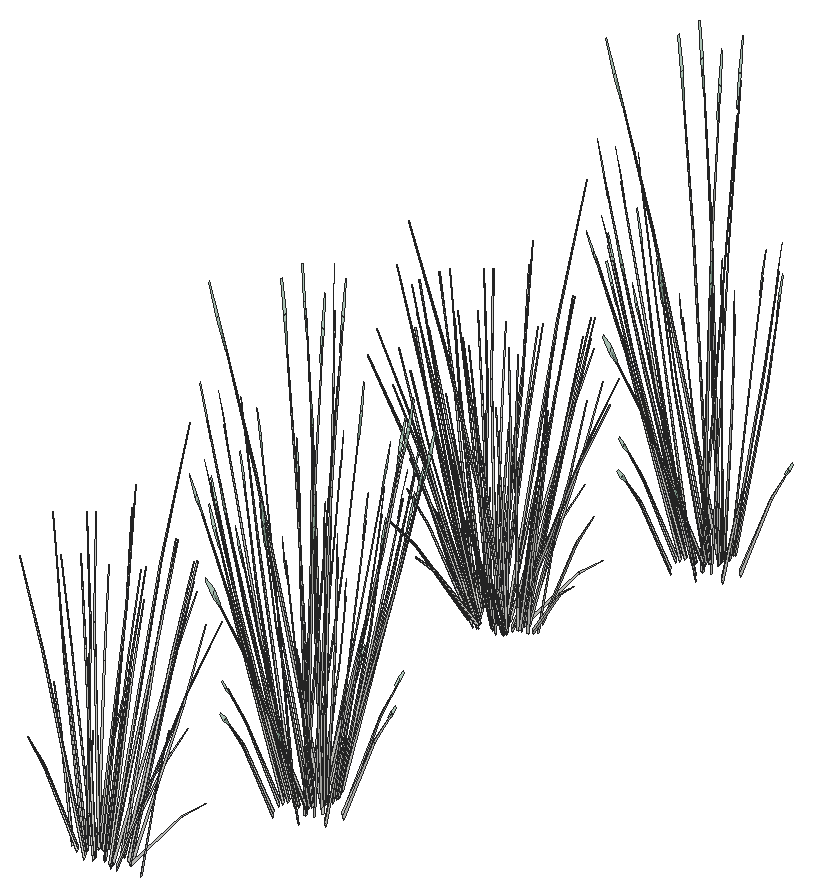
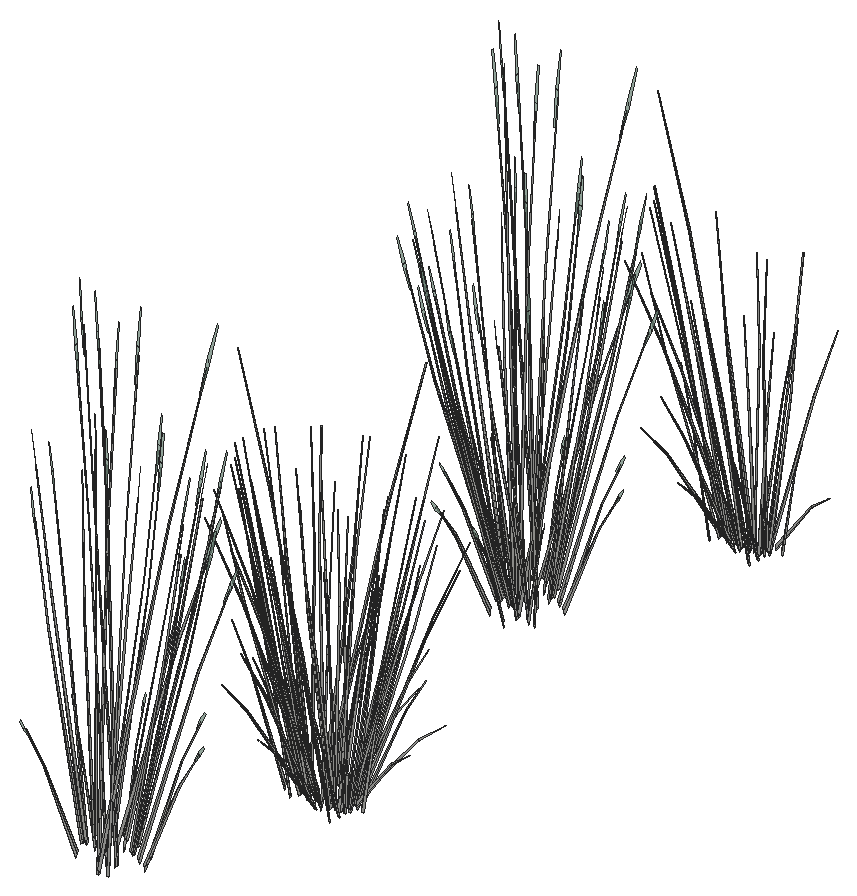
# SketchUp Ruby script. Lengths in inches.
U = 1.inch
M = Sketchup.active_model
def pt(a) = Geom::Point3d.new(a.map { |v| v * U })
def face(e, loops, mat)
  f = e.add_face(loops[0].map { |a| pt(a) })
  loops[1..].each { |l| e.add_face(l.map { |a| pt(a) }).erase! }
  f.material = f.back_material = mat if mat
  f
end
# faces: each face lists its corners as indices into pts; further lists are holes
def faces(e, pts, list, mat = nil) = list.each { |f| face(e, (f[0].is_a?(Array) ? f : [f]).map { |l| l.map { |i| pts[i] } }, mat) }
# xy, xz, yz: faces in a plane at the given z, y or x. An outline is a flat list of corners, or four numbers for a rectangle; further outlines are holes
def ring(l) = l.size == 4 ? [[l[0], l[1]], [l[2], l[1]], [l[2], l[3]], [l[0], l[3]]] : l.each_slice(2).to_a
def flat(e, list, mat, &to3) = list.each { |f| face(e, (f[0].is_a?(Array) ? f : [f]).map { |l| ring(l).map { |u, v| to3.(u, v) } }, mat) }
def xy(e, z, list, mat = nil) = flat(e, list, mat) { |x, y| [x, y, z] }
def xz(e, y, list, mat = nil) = flat(e, list, mat) { |x, z| [x, y, z] }
def yz(e, x, list, mat = nil) = flat(e, list, mat) { |y, z| [x, y, z] }
def lines(e, pts, list) = list.each { |a, b| e.add_line(pt(pts[a]), pt(pts[b])) }
# prism: a flat outline (further loops are holes) pulled along v
def prism(e, loops, v, mat = nil)
  f = face(e, loops, mat); d = Geom::Vector3d.new(v.map { |x| x * U })
  f.pushpull(f.normal.samedirection?(d) ? d.length : -d.length)
end
def box(e, o, s, mat = nil) = prism(e, [[o, [o[0] + s[0], o[1], o[2]], [o[0] + s[0], o[1] + s[1], o[2]], [o[0], o[1] + s[1], o[2]]]], [0, 0, s[2]], mat)
def at(x, y, z, deg = 0) = Geom::Transformation.translation(pt([x, y, z])) * Geom::Transformation.rotation(ORIGIN, Z_AXIS, deg.degrees)
def axes(o, x, y, z) = Geom::Transformation.new([*x, 0, *y, 0, *z, 0, *pt(o).to_a, 1])
def part(name) = M.definitions.add(name)
# library, detail: a bought-in or finely detailed component or shape, given as its bounding box
def library(name, o, s) = part(name).tap { |d| box(d.entities, o, s) }
def detail(e, o, s) = box(e.add_group.entities, o, s)
def put(e, d, t, mat = nil) = e.add_instance(d, t).tap { |i| i.material = mat if mat }
def group(e, t, mat = nil) = e.add_group.tap { |g| g.transformation = t; g.material = mat if mat }.entities
root = M.entities
M.materials.add("LightPink_Translucent").color = [175, 214, 192]
M.materials["LightPink_Translucent"].alpha = 0.75
c1 = part("blade")
p = [[2.15,0.21,22],[0,0.17,0],[0.09,0.45,0],[2.18,0.31,22],[2.29,0.31,22],[0.38,0.45,0],
  [2.48,0.24,33],[2.49,0.24,33],[2.48,0.22,33]]
faces(c1.entities,p,[[0,1,2,3],[4,5,2,3],[6,3,4,7],[8,0,3,6]])
c2 = part("blade with seeds\#1")
put(c2.entities,c1,at(0,0,0))
c3 = part("seeds")
p = [[0.3,-0.1,1.38],[-0.01,-0.03,1.59],[-0.01,-0.03,0.03],[0.14,-0.07,-0.07],[0.29,-0.03,3],[0.15,0.01,3.11]]
faces(c3.entities,p,[[0,1,2,3],[1,0,4,5]],"LightPink_Translucent")
c4 = part("blade with seeds")
put(c4.entities,c1,at(0,0,0))
put(c4.entities,c3,axes([2.4,0.25,30.99],[1.5799,-0.05474,1.17369],[-0.12525,1.92788,0.29478],[-0.07173,-0.02425,1.56792]))
put(root,c2,axes([483.4375,257.72,140.59],[-0.08118,0.04947,1.43516],[0.00691,0.36146,-0.22697],[-0.18608,0.04701,0.1151]))
put(root,c2,axes([488.9,258.875,139.94],[-0.09515,-0.32031,-0.02864],[0.44972,-0.07364,-0.12987],[0.09391,0.02031,0.42837]))
put(root,c2,axes([487.73,258.87,140.85],[0.02662,-0.38751,-0.09976],[0.50399,0.01059,-0.55369],[0.19411,0.02692,0.84132]))
put(root,c2,axes([488.17,258.63,140.59],[0.10664,-0.00644,1.43516],[0.29251,-0.29603,-0.22697],[0.18969,0.03908,0.1151]))
put(root,c2,axes([483.9,258.35,140.6],[-0.12329,-0.35069,0.39379],[0.48364,-0.06086,0.3247],[-0.14254,0.08248,0.81485]))
put(root,c2,axes([483.96,257.86,139.9],[0.17249,-0.0806,1.40588],[0.14522,0.37244,0.11368],[-0.2708,0.08417,0.601]))
put(root,c2,axes([482.53,258.09,140.58],[0.06344,0.01022,1.45516],[0.19627,0.33667,-0.1375],[-0.12987,0.08837,0.25751]))
put(root,c2,axes([483.85,258.41,140.43],[-0.43273,0.05446,-0.29052],[-0.11427,-0.31131,0.37506],[-0.12401,0.08362,0.71765]))
put(root,c2,axes([488.05,258.84,140.43],[0.28286,0.23857,-0.29052],[-0.32298,0.22584,0.37506],[0.1641,0.03436,0.71765]))
put(root,c2,axes([487.94,258.84,140.6],[-0.36656,0.25108,0.39379],[-0.31614,-0.26664,0.3247],[0.17198,0.04631,0.81485]))
put(root,c2,axes([487.07,257.36,140.39],[-0.42958,-0.19798,1.1344],[0.45359,-0.30825,0.48946],[0.1386,0.18577,1.09651]))
put(root,c2,axes([487.04,258.23,139.9],[-0.18466,-0.06565,1.40588],[0.38215,-0.27542,0.11368],[0.23818,0.12424,0.601]))
put(root,c2,axes([483.98,258.2,140.85],[0.45986,0.21011,-0.09976],[-0.26493,0.30427,-0.55369],[-0.12992,0.10577,0.84132]))
put(root,c2,axes([484.6,258.11,139.9],[0.12417,-0.11708,1.40588],[0.31352,0.31602,0.11368],[-0.21504,0.14392,0.601]))
put(root,c2,axes([486.74,259.29,140.85],[0.29624,-0.32616,-0.09976],[0.42901,0.1879,-0.55369],[0.14913,0.09215,0.84132]))
put(root,c2,axes([486.35,259.56,140.58],[0.00147,-0.04613,1.45516],[0.42603,-0.20353,-0.1375],[0.14798,0.07265,0.25751]))
put(root,c2,axes([484.61,259.06,140.6],[-0.354,-0.25999,0.39379],[0.37594,-0.22422,0.3247],[-0.0653,0.12198,0.81485]))
put(root,c2,axes([486.94,259.34,140.6],[-0.49445,0.08745,0.39379],[-0.08581,-0.34303,0.3247],[0.11629,0.1011,0.81485]))
put(root,c2,axes([484.5,258.39,139.9],[0.09256,-0.13097,1.40588],[0.38832,0.27104,0.11368],[-0.17518,0.16893,0.601]))
put(root,c2,axes([484.61,259.13,140.43],[-0.33637,0.20062,-0.29052],[-0.31842,-0.22908,0.37506],[-0.04845,0.11639,0.71765]))
put(root,c2,axes([485.59,259.44,140.6],[-0.36632,0.1295,0.05275],[-0.1793,-0.23615,0.41527],[0.03538,0.1041,0.63322]))
put(root,c2,axes([483.45,259.07,140.59],[-0.01236,0.0754,1.43516],[0.35069,0.26232,-0.22697],[-0.09181,0.12405,0.1151]))
put(root,c2,axes([484.57,258.9,141.15],[0.54637,0.01888,-0.11073],[-0.01493,0.35746,-0.6146],[-0.03795,0.13767,0.93387]))
put(root,c2,axes([485.58,259.3,140.85],[0.48648,-0.17741,-0.09976],[0.23906,0.31487,-0.55369],[0.06419,0.13269,0.84132]))
put(root,c2,axes([484.94,259.04,140.82],[0.35588,0.25603,-0.4653],[-0.37594,0.22422,-0.36041],[-0.05415,0.13008,0.89031]))
put(root,c2,axes([486.28,258.61,139.9],[-0.11364,-0.12234,1.40588],[0.52511,-0.103,0.11368],[0.11868,0.19206,0.601]))
put(root,c2,axes([485.78,259.49,140.43],[-0.14987,0.29303,-0.29052],[-0.43725,-0.08547,0.37506],[0.04009,0.11798,0.71765]))
put(root,c2,axes([485.35,258.67,139.9],[-0.01217,-0.14625,1.40588],[0.52737,0.09702,0.11368],[-0.03262,0.20842,0.601]))
put(root,c2,axes([483.41,259.85,140.58],[0.0564,-0.02301,1.45516],[0.46615,0.15302,-0.1375],[-0.01095,0.12741,0.25751]))
put(root,c2,axes([485.47,260.01,140.59],[0.06302,0.06136,1.43516],[0.50855,0.02411,-0.22697],[0.05114,0.13532,0.1151]))
put(root,c2,axes([484.65,259.42,139.48],[0.01092,-0.19671,1.26617],[0.49126,0.1039,0.17497],[-0.04257,0.20964,0.59789]))
put(root,c4,axes([493.37,274.375,140.21],[0.06442,0.13585,1.61128],[-0.4498,0.04685,0.1261],[-0.05969,-0.29426,0.57588]))
put(root,c4,axes([494.09,273.93,141.7],[0.01072,-0.47777,-0.64651],[0.45152,0.03209,0.07802],[0.04765,-0.2024,0.91455]))
put(root,c4,axes([493.3125,273.17,141.29],[0.12423,-0.3972,-0.32227],[0.36244,0.11585,0.41605],[-0.03323,-0.15992,0.79608]))
put(root,c4,axes([493.125,273.4375,141.43],[-0.40508,-0.12948,-0.465],[0.13885,-0.44393,-0.36018],[-0.03714,-0.17873,0.88973]))
put(root,c4,axes([494,273.78,141.43],[-0.29499,-0.34704,-0.465],[0.31162,-0.30393,-0.36018],[0.04488,-0.17633,0.88973]))
put(root,c4,axes([491.39,272.5625,139.6875],[0.20183,0.19918,1.04523],[-0.31952,0.0786,0.76796],[-0.05721,-0.14394,0.23022]))
put(root,c4,axes([494.28,273.65,141.29],[0.27882,-0.27194,-0.32227],[0.26394,0.31051,0.41605],[0.04016,-0.15777,0.79608]))
put(root,c4,axes([492.27,273.3125,141.29],[-0.06364,-0.41603,-0.32227],[0.36383,-0.10985,0.41605],[-0.09772,-0.11922,0.79608]))
put(root,c4,axes([493.61,272.99,139.6875],[0.03187,0.30513,1.04523],[-0.28077,-0.19355,0.76796],[0.04212,-0.15079,0.23022]))
put(root,c4,axes([492.22,273.65,141.43],[-0.40663,0.12278,-0.465],[-0.07113,-0.46497,-0.36018],[-0.10922,-0.13325,0.88973]))
put(root,c4,axes([494.625,274.76,141.7],[0.21525,-0.40754,-0.64651],[0.37719,0.28963,0.07802],[0.12852,-0.14765,0.91455]))
put(root,c4,axes([494.61,274.57,141.43],[-0.10586,-0.47162,-0.465],[0.4009,-0.0825,-0.36018],[0.11489,-0.12667,0.88973]))
put(root,c4,axes([494.91,274.625,141.29],[0.3587,-0.07382,-0.32227],[0.09472,0.42197,0.41605],[0.10279,-0.11334,0.79608]))
put(root,c4,axes([491.42,274.04,141.29],[-0.23447,-0.32338,-0.32227],[0.26773,-0.30612,0.41605],[-0.13603,-0.04658,0.79608]))
put(root,c4,axes([492.19,275.74,140.2],[-0.17958,0.41302,1.37647],[-0.38687,-0.40462,0.54432],[0.22929,-0.18124,1.15394]))
put(root,c4,axes([495.45,274.16,139.6875],[-0.155,0.24931,1.04523],[-0.09317,-0.36309,0.76796],[0.11912,-0.07769,0.23022]))
put(root,c4,axes([491.67,274.26,142.03],[-0.41193,-0.01244,-0.71763],[0.02767,-0.52368,0.0866],[-0.17451,-0.05527,1.01516]))
put(root,c4,axes([490.51,274.25,139.6875],[0.2648,-0.01237,1.04523],[-0.18886,0.30908,0.76796],[-0.12621,-0.06079,0.23022]))
put(root,c4,axes([491.09,274.08,140.23],[0.22989,0.0105,1.40454],[-0.12143,0.4723,0.19409],[-0.24501,-0.04092,0.66323]))
put(root,c4,axes([491.54,274.37,141.72],[-0.29922,0.34214,-0.51615],[-0.26205,-0.36143,-0.3998],[-0.15203,-0.05206,0.9876]))
put(root,c4,axes([493.05,276.38,139.76],[0.4193,-0.01306,1.28558],[-0.10869,0.59089,0.54432],[-0.22943,-0.13975,1.21348]))
put(root,c4,axes([494.8,275.62,141.43],[0.11164,-0.46982,-0.465],[0.38276,0.16104,-0.36018],[0.1541,-0.04308,0.88973]))
put(root,c4,axes([492.79,275.03,139.64],[-0.40128,-0.23189,0.40713],[0.19312,-0.48183,-0.19594],[0.0925,0,1.30716]))
put(root,c4,axes([494.73,275.79,141.7],[0.3621,-0.22811,-0.64651],[0.2018,0.46957,0.07802],[0.17496,-0.05334,0.91455]))
put(root,c4,axes([492.61,276.15,139.64],[0.02749,0.519,0.40713],[-0.45634,0.04694,-0.19594],[-0.04625,-0.09291,1.30716]))
put(root,c4,axes([495.04,275.84,141.29],[0.34247,0.14409,-0.32227],[-0.09989,0.42037,0.41605],[0.13788,-0.03855,0.79608]))
put(root,c4,axes([491.01,275.17,141.29],[-0.34247,-0.14409,-0.32227],[0.09989,-0.42037,0.41605],[-0.13788,0.03855,0.79608]))
put(root,c4,axes([493.35,275.15,139.64],[-0.02749,-0.519,0.40713],[0.45634,-0.04694,-0.19594],[0.04625,0.09291,1.30716]))
put(root,c4,axes([491.32,275.21,141.7],[-0.3621,0.22811,-0.64651],[-0.2018,-0.46957,0.07802],[-0.17496,0.05334,0.91455]))
put(root,c4,axes([495.76,275.91,139.6875],[-0.25968,0.06131,1.04523],[0.14383,-0.34012,0.76796],[0.13297,0.0366,0.23022]))
put(root,c4,axes([493.17,276.27,139.64],[0.40128,0.23189,0.40713],[-0.19312,0.48183,-0.19594],[-0.0925,0,1.30716]))
put(root,c4,axes([491.25,275.38,141.43],[-0.11164,0.46982,-0.465],[-0.38276,-0.16104,-0.36018],[-0.1541,0.04308,0.88973]))
put(root,c4,axes([493.54,275.77,139.64],[0.37379,-0.28711,0.40713],[0.26322,0.43489,-0.19594],[-0.04625,0.09291,1.30716]))
put(root,c4,axes([494.51,276.64,141.43],[0.29922,-0.34214,-0.465],[0.26205,0.36143,-0.36018],[0.15203,0.05206,0.88973]))
put(root,c4,axes([494.375,276.74,141.7],[0.41193,0.01244,-0.64651],[-0.02767,0.52368,0.07802],[0.17451,0.05527,0.91455]))
put(root,c4,axes([494.62,276.96,141.29],[0.23447,0.32338,-0.32227],[-0.26773,0.30612,0.41605],[0.13603,0.04658,0.79608]))
put(root,c4,axes([491.61,277.04,139.6875],[0.12805,-0.2691,1.04523],[0.13011,0.34747,0.76796],[-0.11021,0.09372,0.23022]))
put(root,c4,axes([491.02,277.08,139.6],[0.01397,-0.30649,0.95605],[0.29664,0.2024,0.52785],[-0.10539,0.12108,0.74993]))
put(root,c4,axes([491.43,276.43,141.43],[0.10586,0.47162,-0.465],[-0.4009,0.0825,-0.36018],[-0.11489,0.12667,0.88973]))
put(root,c4,axes([493.82,277.35,141.43],[0.40663,-0.12278,-0.465],[0.07113,0.46497,-0.36018],[0.10922,0.13325,0.88973]))
put(root,c4,axes([491.72,278.16,140.75],[0.37435,-0.09148,-0.03177],[0.08606,0.43236,-0.14407],[-0.02373,0.09029,0.47519]))
put(root,c4,axes([494.63,277.92,139.6875],[-0.2267,-0.15919,1.04523],[0.30457,-0.13683,0.76796],[0.07632,0.13148,0.23022]))
put(root,c4,axes([493.78,277.69,141.29],[0.06364,0.41603,-0.32227],[-0.36383,0.10985,0.41605],[0.09772,0.11922,0.79608]))
put(root,c4,axes([493.66,277.36,141.7],[0.35138,0.24965,-0.64651],[-0.24972,0.43748,0.07802],[0.12731,0.14906,0.91455]))
put(root,c4,axes([491.77,277.36,141.29],[-0.27882,0.27194,-0.32227],[-0.26394,-0.31051,0.41605],[-0.04016,0.15777,0.79608]))
put(root,c4,axes([492.92,277.5625,141.43],[0.40508,0.12948,-0.465],[-0.13885,0.44393,-0.36018],[0.03714,0.17873,0.88973]))
put(root,c4,axes([492.66,278.68,139.6875],[-0.07352,-0.2953,1.04523],[0.30384,0.139,0.76796],[-0.02079,0.15666,0.23022]))
put(root,c4,axes([492.73,277.84,141.29],[-0.12423,0.3972,-0.32227],[-0.36244,-0.11585,0.41605],[0.03323,0.15992,0.79608]))
put(root,c4,axes([491.95,277.07,141.7],[-0.01072,0.47777,-0.64651],[-0.45152,-0.03209,0.07802],[-0.04765,0.2024,0.91455]))
put(root,c4,axes([492.77,277.48,141.7],[0.19668,0.41997,-0.64651],[-0.40486,0.23405,0.07802],[0.04599,0.20292,0.91455]))
put(root,c2,axes([485.03,306.2,139.9],[0.11364,0.12234,1.40588],[-0.52511,0.103,0.11368],[-0.11868,-0.19206,0.601]))
put(root,c2,axes([485.9,305.39,140.59],[-0.07604,-0.05342,1.43516],[-0.50744,0.03387,-0.22697],[-0.08099,-0.12778,0.1151]))
put(root,c2,axes([488.07,305.77,140.58],[-0.05049,0.0291,1.45516],[-0.49465,-0.09819,-0.1375],[-0.01791,-0.12701,0.25751]))
put(root,c2,axes([488.18,306.05,140.59],[-0.0048,-0.07584,1.43516],[-0.40531,-0.21918,-0.22697],[0.06266,-0.13286,0.1151]))
put(root,c2,axes([486.8,306.42,139.9],[-0.09256,0.13097,1.40588],[-0.38832,-0.27104,0.11368],[0.17518,-0.16893,0.601]))
put(root,c2,axes([486.47,306.03,140.43],[0.14987,-0.29303,-0.29052],[0.43725,0.08547,0.37506],[-0.04009,-0.11798,0.71765]))
put(root,c2,axes([485.375,305.22,140.58],[-0.00927,0.04567,1.45516],[-0.45742,0.16576,-0.1375],[-0.1346,-0.08473,0.25751]))
put(root,c2,axes([486.67,306.22,140.85],[-0.48648,0.17741,-0.09976],[-0.23906,-0.31487,-0.55369],[-0.06419,-0.13269,0.84132]))
put(root,c2,axes([486.53,306.1,140.6],[0.48986,0.09962,0.39379],[-0.16751,0.3275,0.3247],[-0.02944,-0.12879,0.81485]))
put(root,c2,axes([487.68,306.61,140.85],[-0.54637,-0.01888,-0.09976],[0.01493,-0.35746,-0.55369],[0.03795,-0.13767,0.84132]))
put(root,c2,axes([485.21,306.14,140.43],[-0.07678,-0.30692,-0.29052],[0.43892,-0.08104,0.37506],[-0.11789,-0.08795,0.71765]))
put(root,c2,axes([487.64,306.38,140.43],[0.33637,-0.20062,-0.29052],[0.31842,0.22908,0.37506],[0.04845,-0.11639,0.71765]))
put(root,c2,axes([484.27,306.58,139.9],[0.18466,0.06565,1.40588],[-0.38215,0.27542,0.11368],[-0.23818,-0.12424,0.601]))
put(root,c2,axes([485.5,306.08,141.17],[-0.33178,0.3653,-0.11173],[-0.48049,-0.21045,-0.62013],[-0.16702,-0.10321,0.94228]))
put(root,c2,axes([487.64,306.46,140.6],[0.354,0.25999,0.39379],[-0.37594,0.22422,0.3247],[0.0653,-0.12198,0.81485]))
put(root,c2,axes([484.23,305.98,140.59],[-0.10696,-0.00269,1.43516],[-0.34054,0.26896,-0.22697],[-0.1817,-0.05496,0.1151]))
put(root,c2,axes([488.27,307.32,140.85],[-0.45986,-0.21011,-0.09976],[0.26493,-0.30427,-0.55369],[0.12992,-0.10577,0.84132]))
put(root,c2,axes([489.41,307.23,140.58],[-0.06493,-0.00289,1.45516],[-0.26964,-0.31009,-0.1375],[0.10828,-0.10196,0.25751]))
put(root,c2,axes([486.375,308.47,139.45],[0.4296,0.15365,1.24087],[-0.42086,0.33102,0.4907],[-0.18851,-0.19619,1.04025]))
put(root,c2,axes([484.2,306.68,140.43],[-0.28286,-0.23857,-0.29052],[0.32298,-0.22584,0.37506],[-0.1641,-0.03436,0.71765]))
put(root,c2,axes([488.4,307.11,140.43],[0.43273,-0.05446,-0.29052],[0.11427,0.31131,0.37506],[0.12401,-0.08362,0.71765]))
put(root,c2,axes([488.35,307.17,140.6],[0.12329,0.35069,0.39379],[-0.48364,0.06086,0.3247],[0.14254,-0.08248,0.81485]))
put(root,c2,axes([489.65,307.6,140.59],[0.06898,-0.05804,1.43516],[-0.0883,-0.35603,-0.22697],[0.17309,-0.0675,0.1151]))
put(root,c2,axes([483.82,306.21,140.58],[0.03685,0.03803,1.45516],[-0.17767,0.34183,-0.1375],[-0.17994,0.00247,0.25751]))
put(root,c2,axes([484.52,306.65,140.85],[-0.02662,0.38751,-0.09976],[-0.50399,-0.01059,-0.55369],[-0.19411,-0.02692,0.84132]))
put(root,c2,axes([488.29,308.14,140.85],[-0.25013,-0.34504,-0.09976],[0.44394,-0.16956,-0.55369],[0.18708,-0.04552,0.84132]))
put(root,c2,axes([483.88,307.18,139.9],[0.2062,-0.00863,1.40588],[-0.13679,0.37404,0.11368],[-0.29386,-0.02314,0.601]))
put(root,c2,axes([483.79,307.47,140.6],[0.14045,-0.34743,0.39379],[0.46175,0.1188,0.3247],[-0.18159,0.02088,0.81485]))
put(root,c2,axes([483.7,307.51,140.43],[-0.41315,-0.1063,-0.29052],[0.1205,-0.31012,0.37506],[-0.16634,0.02844,0.71765]))
put(root,c2,axes([488.55,308,140.43],[0.41315,0.1063,-0.29052],[-0.1205,0.31012,0.37506],[0.16634,-0.02844,0.71765]))
put(root,c2,axes([487.43,307.62,139.9],[-0.2062,0.00863,1.40588],[0.13679,-0.37404,0.11368],[0.29386,0.02314,0.601]))
put(root,c2,axes([488.46,308.04,140.6],[-0.14045,0.34743,0.39379],[-0.46175,-0.1188,0.3247],[0.18159,-0.02088,0.81485]))
put(root,c2,axes([483.96,307.37,140.85],[0.25013,0.34504,-0.09976],[-0.44394,0.16956,-0.55369],[-0.18708,0.04552,0.84132]))
put(root,c2,axes([489.29,309.16,140.58],[-0.04495,-0.03336,1.45516],[0.09833,-0.35758,-0.1375],[0.17707,-0.02285,0.25751]))
put(root,c2,axes([483.4375,307.71,140.59],[-0.08118,0.04947,1.43516],[0.00691,0.36146,-0.22697],[-0.18608,0.04701,0.1151]))
put(root,c2,axes([488.9,308.86,139.94],[-0.09515,-0.32031,-0.02864],[0.44972,-0.07364,-0.12987],[0.09391,0.02031,0.42837]))
put(root,c2,axes([487.73,308.85,140.85],[0.02662,-0.38751,-0.09976],[0.50399,0.01059,-0.55369],[0.19411,0.02692,0.84132]))
put(root,c2,axes([488.17,308.62,140.59],[0.10664,-0.00644,1.43516],[0.29251,-0.29603,-0.22697],[0.18969,0.03908,0.1151]))
put(root,c2,axes([483.9,308.33,140.6],[-0.12329,-0.35069,0.39379],[0.48364,-0.06086,0.3247],[-0.14254,0.08248,0.81485]))
put(root,c2,axes([483.96,307.84,139.9],[0.17249,-0.0806,1.40588],[0.14522,0.37244,0.11368],[-0.2708,0.08417,0.601]))
put(root,c2,axes([482.53,308.08,140.58],[0.06344,0.01022,1.45516],[0.19627,0.33667,-0.1375],[-0.12987,0.08837,0.25751]))
put(root,c2,axes([483.85,308.4,140.43],[-0.43273,0.05446,-0.29052],[-0.11427,-0.31131,0.37506],[-0.12401,0.08362,0.71765]))
put(root,c2,axes([488.05,308.83,140.43],[0.28286,0.23857,-0.29052],[-0.32298,0.22584,0.37506],[0.1641,0.03436,0.71765]))
put(root,c2,axes([487.94,308.83,140.6],[-0.36656,0.25108,0.39379],[-0.31614,-0.26664,0.3247],[0.17198,0.04631,0.81485]))
put(root,c2,axes([487.07,307.35,140.39],[-0.42958,-0.19798,1.1344],[0.45359,-0.30825,0.48946],[0.1386,0.18577,1.09651]))
put(root,c2,axes([487.04,308.22,139.9],[-0.18466,-0.06565,1.40588],[0.38215,-0.27542,0.11368],[0.23818,0.12424,0.601]))
put(root,c2,axes([483.98,308.1875,140.85],[0.45986,0.21011,-0.09976],[-0.26493,0.30427,-0.55369],[-0.12992,0.10577,0.84132]))
put(root,c2,axes([484.6,308.09,139.9],[0.12417,-0.11708,1.40588],[0.31352,0.31602,0.11368],[-0.21504,0.14392,0.601]))
put(root,c2,axes([486.74,309.28,140.85],[0.29624,-0.32616,-0.09976],[0.42901,0.1879,-0.55369],[0.14913,0.09215,0.84132]))
put(root,c2,axes([486.35,309.55,140.58],[0.00147,-0.04613,1.45516],[0.42603,-0.20353,-0.1375],[0.14798,0.07265,0.25751]))
put(root,c2,axes([484.61,309.04,140.6],[-0.354,-0.25999,0.39379],[0.37594,-0.22422,0.3247],[-0.0653,0.12198,0.81485]))
put(root,c2,axes([486.94,309.33,140.6],[-0.49445,0.08745,0.39379],[-0.08581,-0.34303,0.3247],[0.11629,0.1011,0.81485]))
put(root,c2,axes([484.5,308.38,139.9],[0.09256,-0.13097,1.40588],[0.38832,0.27104,0.11368],[-0.17518,0.16893,0.601]))
put(root,c2,axes([484.61,309.12,140.43],[-0.33637,0.20062,-0.29052],[-0.31842,-0.22908,0.37506],[-0.04845,0.11639,0.71765]))
put(root,c2,axes([483.45,309.0625,140.59],[-0.01236,0.0754,1.43516],[0.35069,0.26232,-0.22697],[-0.09181,0.12405,0.1151]))
put(root,c2,axes([484.57,308.89,141.15],[0.54637,0.01888,-0.11073],[-0.01493,0.35746,-0.6146],[-0.03795,0.13767,0.93387]))
put(root,c2,axes([485.58,309.29,140.85],[0.48648,-0.17741,-0.09976],[0.23906,0.31487,-0.55369],[0.06419,0.13269,0.84132]))
put(root,c2,axes([484.94,309.03,140.82],[0.35588,0.25603,-0.4653],[-0.37594,0.22422,-0.36041],[-0.05415,0.13008,0.89031]))
put(root,c2,axes([486.28,308.6,139.9],[-0.11364,-0.12234,1.40588],[0.52511,-0.103,0.11368],[0.11868,0.19206,0.601]))
put(root,c2,axes([485.78,309.47,140.43],[-0.14987,0.29303,-0.29052],[-0.43725,-0.08547,0.37506],[0.04009,0.11798,0.71765]))
put(root,c2,axes([485.35,308.66,139.9],[-0.01217,-0.14625,1.40588],[0.52737,0.09702,0.11368],[-0.03262,0.20842,0.601]))
put(root,c2,axes([483.41,309.83,140.58],[0.0564,-0.02301,1.45516],[0.46615,0.15302,-0.1375],[-0.01095,0.12741,0.25751]))
put(root,c2,axes([485.47,309.99,140.59],[0.06302,0.06136,1.43516],[0.50855,0.02411,-0.22697],[0.05114,0.13532,0.1151]))
put(root,c2,axes([484.65,309.41,139.48],[0.01092,-0.19671,1.26617],[0.49126,0.1039,0.17497],[-0.04257,0.20964,0.59789]))
put(root,c4,axes([493.37,324.36,140.21],[0.06442,0.13585,1.61128],[-0.4498,0.04685,0.1261],[-0.05969,-0.29426,0.57588]))
put(root,c4,axes([494.09,323.92,141.7],[0.01072,-0.47777,-0.64651],[0.45152,0.03209,0.07802],[0.04765,-0.2024,0.91455]))
put(root,c4,axes([493.3125,323.15,141.29],[0.12423,-0.3972,-0.32227],[0.36244,0.11585,0.41605],[-0.03323,-0.15992,0.79608]))
put(root,c4,axes([493.125,323.43,141.43],[-0.40508,-0.12948,-0.465],[0.13885,-0.44393,-0.36018],[-0.03714,-0.17873,0.88973]))
put(root,c4,axes([494,323.76,141.43],[-0.29499,-0.34704,-0.465],[0.31162,-0.30393,-0.36018],[0.04488,-0.17633,0.88973]))
put(root,c4,axes([491.39,322.55,139.6875],[0.20183,0.19918,1.04523],[-0.31952,0.0786,0.76796],[-0.05721,-0.14394,0.23022]))
put(root,c4,axes([494.28,323.63,141.29],[0.27882,-0.27194,-0.32227],[0.26394,0.31051,0.41605],[0.04016,-0.15777,0.79608]))
put(root,c4,axes([492.27,323.3,141.29],[-0.06364,-0.41603,-0.32227],[0.36383,-0.10985,0.41605],[-0.09772,-0.11922,0.79608]))
put(root,c4,axes([493.61,322.98,139.6875],[0.03187,0.30513,1.04523],[-0.28077,-0.19355,0.76796],[0.04212,-0.15079,0.23022]))
put(root,c4,axes([492.22,323.64,141.43],[-0.40663,0.12278,-0.465],[-0.07113,-0.46497,-0.36018],[-0.10922,-0.13325,0.88973]))
put(root,c4,axes([494.625,324.75,141.7],[0.21525,-0.40754,-0.64651],[0.37719,0.28963,0.07802],[0.12852,-0.14765,0.91455]))
put(root,c4,axes([494.61,324.5625,141.43],[-0.10586,-0.47162,-0.465],[0.4009,-0.0825,-0.36018],[0.11489,-0.12667,0.88973]))
put(root,c4,axes([494.91,324.61,141.29],[0.3587,-0.07382,-0.32227],[0.09472,0.42197,0.41605],[0.10279,-0.11334,0.79608]))
put(root,c4,axes([491.42,324.03,141.29],[-0.23447,-0.32338,-0.32227],[0.26773,-0.30612,0.41605],[-0.13603,-0.04658,0.79608]))
put(root,c4,axes([492.19,325.73,140.2],[-0.17958,0.41302,1.37647],[-0.38687,-0.40462,0.54432],[0.22929,-0.18124,1.15394]))
put(root,c4,axes([495.45,324.15,139.6875],[-0.155,0.24931,1.04523],[-0.09317,-0.36309,0.76796],[0.11912,-0.07769,0.23022]))
put(root,c4,axes([491.67,324.25,142.03],[-0.41193,-0.01244,-0.71763],[0.02767,-0.52368,0.0866],[-0.17451,-0.05527,1.01516]))
put(root,c4,axes([490.51,324.24,139.6875],[0.2648,-0.01237,1.04523],[-0.18886,0.30908,0.76796],[-0.12621,-0.06079,0.23022]))
put(root,c4,axes([491.09,324.07,140.23],[0.22989,0.0105,1.40454],[-0.12143,0.4723,0.19409],[-0.24501,-0.04092,0.66323]))
put(root,c4,axes([491.54,324.35,141.72],[-0.29922,0.34214,-0.51615],[-0.26205,-0.36143,-0.3998],[-0.15203,-0.05206,0.9876]))
put(root,c4,axes([493.05,326.37,139.76],[0.4193,-0.01306,1.28558],[-0.10869,0.59089,0.54432],[-0.22943,-0.13975,1.21348]))
put(root,c4,axes([494.8,325.61,141.43],[0.11164,-0.46982,-0.465],[0.38276,0.16104,-0.36018],[0.1541,-0.04308,0.88973]))
put(root,c4,axes([492.79,325.01,139.64],[-0.40128,-0.23189,0.40713],[0.19312,-0.48183,-0.19594],[0.0925,0,1.30716]))
put(root,c4,axes([494.73,325.78,141.7],[0.3621,-0.22811,-0.64651],[0.2018,0.46957,0.07802],[0.17496,-0.05334,0.91455]))
put(root,c4,axes([492.61,326.13,139.64],[0.02749,0.519,0.40713],[-0.45634,0.04694,-0.19594],[-0.04625,-0.09291,1.30716]))
put(root,c4,axes([495.04,325.82,141.29],[0.34247,0.14409,-0.32227],[-0.09989,0.42037,0.41605],[0.13788,-0.03855,0.79608]))
put(root,c4,axes([491.01,325.15,141.29],[-0.34247,-0.14409,-0.32227],[0.09989,-0.42037,0.41605],[-0.13788,0.03855,0.79608]))
put(root,c4,axes([493.35,325.14,139.64],[-0.02749,-0.519,0.40713],[0.45634,-0.04694,-0.19594],[0.04625,0.09291,1.30716]))
put(root,c4,axes([491.32,325.2,141.7],[-0.3621,0.22811,-0.64651],[-0.2018,-0.46957,0.07802],[-0.17496,0.05334,0.91455]))
put(root,c4,axes([495.76,325.9,139.6875],[-0.25968,0.06131,1.04523],[0.14383,-0.34012,0.76796],[0.13297,0.0366,0.23022]))
put(root,c4,axes([493.17,326.26,139.64],[0.40128,0.23189,0.40713],[-0.19312,0.48183,-0.19594],[-0.0925,0,1.30716]))
